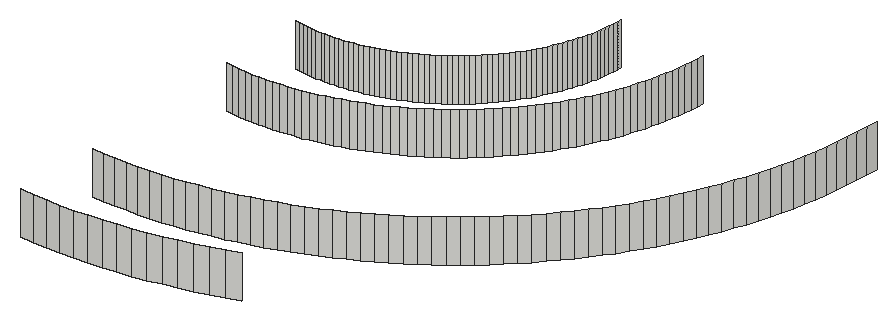
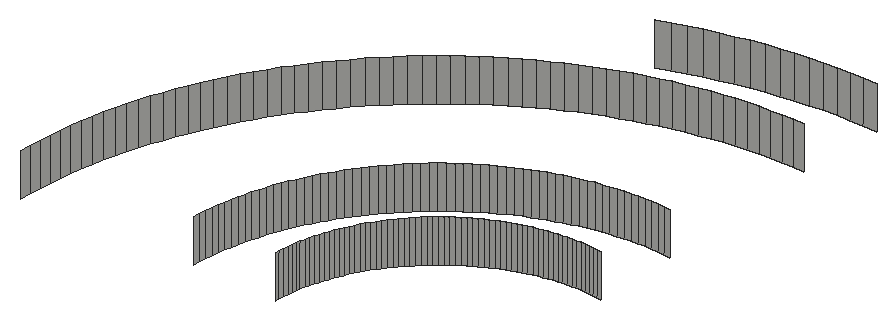
# SketchUp Ruby script. Lengths in inches.
U = 1.inch
M = Sketchup.active_model
def pt(a) = Geom::Point3d.new(a.map { |v| v * U })
def face(e, loops, mat)
  f = e.add_face(loops[0].map { |a| pt(a) })
  loops[1..].each { |l| e.add_face(l.map { |a| pt(a) }).erase! }
  f.material = f.back_material = mat if mat
  f
end
# faces: each face lists its corners as indices into pts; further lists are holes
def faces(e, pts, list, mat = nil) = list.each { |f| face(e, (f[0].is_a?(Array) ? f : [f]).map { |l| l.map { |i| pts[i] } }, mat) }
# xy, xz, yz: faces in a plane at the given z, y or x. An outline is a flat list of corners, or four numbers for a rectangle; further outlines are holes
def ring(l) = l.size == 4 ? [[l[0], l[1]], [l[2], l[1]], [l[2], l[3]], [l[0], l[3]]] : l.each_slice(2).to_a
def flat(e, list, mat, &to3) = list.each { |f| face(e, (f[0].is_a?(Array) ? f : [f]).map { |l| ring(l).map { |u, v| to3.(u, v) } }, mat) }
def xy(e, z, list, mat = nil) = flat(e, list, mat) { |x, y| [x, y, z] }
def xz(e, y, list, mat = nil) = flat(e, list, mat) { |x, z| [x, y, z] }
def yz(e, x, list, mat = nil) = flat(e, list, mat) { |y, z| [x, y, z] }
def lines(e, pts, list) = list.each { |a, b| e.add_line(pt(pts[a]), pt(pts[b])) }
# prism: a flat outline (further loops are holes) pulled along v
def prism(e, loops, v, mat = nil)
  f = face(e, loops, mat); d = Geom::Vector3d.new(v.map { |x| x * U })
  f.pushpull(f.normal.samedirection?(d) ? d.length : -d.length)
end
def box(e, o, s, mat = nil) = prism(e, [[o, [o[0] + s[0], o[1], o[2]], [o[0] + s[0], o[1] + s[1], o[2]], [o[0], o[1] + s[1], o[2]]]], [0, 0, s[2]], mat)
def at(x, y, z, deg = 0) = Geom::Transformation.translation(pt([x, y, z])) * Geom::Transformation.rotation(ORIGIN, Z_AXIS, deg.degrees)
def axes(o, x, y, z) = Geom::Transformation.new([*x, 0, *y, 0, *z, 0, *pt(o).to_a, 1])
def part(name) = M.definitions.add(name)
# library, detail: a bought-in or finely detailed component or shape, given as its bounding box
def library(name, o, s) = part(name).tap { |d| box(d.entities, o, s) }
def detail(e, o, s) = box(e.add_group.entities, o, s)
def put(e, d, t, mat = nil) = e.add_instance(d, t).tap { |i| i.material = mat if mat }
def group(e, t, mat = nil) = e.add_group.tap { |g| g.transformation = t; g.material = mat if mat }.entities
root = M.entities
xz(root,301.26,[[905.35,111.3125,905.98,117.3125],[905.98,111.3125,906.61,117.3125]])
p = [[904.09,253.28,117.3125],[902.21,253.35,117.3125],[902.21,253.35,111.3125],[904.09,253.28,111.3125],[905.98,253.26,117.3125],[905.98,253.26,111.3125],
  [907.86,253.28,117.3125],[907.86,253.28,111.3125],[909.75,253.35,117.3125],[909.75,253.35,111.3125],[911.63,253.48,117.3125],[911.63,253.48,111.3125],
  [913.5,253.65,117.3125],[913.5,253.65,111.3125],[915.375,253.87,117.3125],[915.375,253.87,111.3125],[917.24,254.14,117.3125],[917.24,254.14,111.3125],
  [919.1,254.46,117.3125],[919.1,254.46,111.3125],[920.95,254.83,117.3125],[920.95,254.83,111.3125],[922.79,255.25,117.3125],[922.79,255.25,111.3125],
  [924.61,255.71,117.3125],[924.61,255.71,111.3125],[926.43,256.22,117.3125],[926.43,256.22,111.3125],[928.23,256.78,117.3125],[928.23,256.78,111.3125],
  [930.01,257.39,117.3125],[930.01,257.39,111.3125],[902.84,265.34,117.3125],[904.41,265.28,117.3125],[904.41,265.28,111.3125],[902.84,265.34,111.3125],
  [905.98,265.26,117.3125],[905.98,265.26,111.3125],[907.55,265.28,117.3125],[907.55,265.28,111.3125],[909.12,265.34,117.3125],[909.12,265.34,111.3125],
  [910.6875,265.44,117.3125],[910.6875,265.44,111.3125],[912.25,265.58,117.3125],[912.25,265.58,111.3125],[913.81,265.77,117.3125],[913.81,265.77,111.3125],
  [915.36,265.99,117.3125],[915.36,265.99,111.3125],[916.91,266.26,117.3125],[916.91,266.26,111.3125],[918.45,266.57,117.3125],[918.45,266.57,111.3125],
  [919.99,266.91,117.3125],[919.99,266.91,111.3125],[921.51,267.3,117.3125],[921.51,267.3,111.3125],[923.02,267.73,117.3125],[923.02,267.73,111.3125],
  [924.52,268.19,117.3125],[924.52,268.19,111.3125],[926.01,268.7,117.3125],[926.01,268.7,111.3125],[927.48,269.24,117.3125],[927.48,269.24,111.3125],
  [928.94,269.82,117.3125],[928.94,269.82,111.3125],[930.38,270.44,117.3125],[930.38,270.44,111.3125],[931.81,271.1,117.3125],[931.81,271.1,111.3125],
  [933.22,271.8,117.3125],[933.22,271.8,111.3125],[934.61,272.53,117.3125],[934.61,272.53,111.3125],[935.98,273.29,117.3125],[935.98,273.29,111.3125],
  [937.33,274.1,117.3125],[937.33,274.1,111.3125],[938.66,274.9375,117.3125],[938.66,274.9375,111.3125],[939.96,275.81,117.3125],[939.96,275.81,111.3125],
  [941.25,276.72,117.3125],[941.25,276.72,111.3125],[942.5,277.66,117.3125],[942.5,277.66,111.3125],[943.74,278.63,117.3125],[943.74,278.63,111.3125],
  [944.95,279.63,117.3125],[944.95,279.63,111.3125],[946.125,280.67,117.3125],[946.125,280.67,111.3125],[947.28,281.73,117.3125],[947.28,281.73,111.3125],
  [948.41,282.83,117.3125],[948.41,282.83,111.3125],[949.5,283.95,117.3125],[949.5,283.95,111.3125],[950.57,285.11,117.3125],[950.57,285.11,111.3125],
  [951.6,286.29,117.3125],[951.6,286.29,111.3125],[952.61,287.5,117.3125],[952.61,287.5,111.3125],[953.58,288.73,117.3125],[953.58,288.73,111.3125],
  [954.52,289.99,117.3125],[954.52,289.99,111.3125],[904.09,289.31,117.3125],[903.15,289.37,117.3125],[903.15,289.37,111.3125],[904.09,289.31,111.3125],
  [905.04,289.27,117.3125],[905.04,289.27,111.3125],[905.98,289.26,117.3125],[905.98,289.26,111.3125],[906.92,289.27,117.3125],[906.92,289.27,111.3125],
  [907.86,289.31,117.3125],[907.86,289.31,111.3125],[908.8,289.37,117.3125],[908.8,289.37,111.3125],[902.22,289.45,117.3125],[902.22,289.45,111.3125],
  [909.74,289.45,117.3125],[909.74,289.45,111.3125],[910.68,289.5625,117.3125],[910.68,289.5625,111.3125],[911.61,289.7,117.3125],[911.61,289.7,111.3125],
  [912.54,289.86,117.3125],[912.54,289.86,111.3125],[913.46,290.04,117.3125],[913.46,290.04,111.3125],[914.38,290.25,117.3125],[914.38,290.25,111.3125],
  [955.43,291.27,117.3125],[955.43,291.27,111.3125],[915.3,290.48,117.3125],[915.3,290.48,111.3125],[916.2,290.74,117.3125],[916.2,290.74,111.3125],
  [917.1,291.02,117.3125],[917.1,291.02,111.3125],[918,291.32,117.3125],[918,291.32,111.3125],[918.88,291.65,117.3125],[918.88,291.65,111.3125],
  [956.3,292.58,117.3125],[956.3,292.58,111.3125],[919.76,292,117.3125],[919.76,292,111.3125],[920.62,292.37,117.3125],[920.62,292.37,111.3125],
  [921.48,292.76,117.3125],[921.48,292.76,111.3125],[957.14,293.91,117.3125],[957.14,293.91,111.3125],[922.32,293.18,117.3125],[922.32,293.18,111.3125],
  [923.16,293.62,117.3125],[923.16,293.62,111.3125],[923.98,294.08,117.3125],[923.98,294.08,111.3125],[957.94,295.26,117.3125],[957.94,295.26,111.3125],
  [924.79,294.5625,117.3125],[924.79,294.5625,111.3125],[925.59,295.0625,117.3125],[925.59,295.0625,111.3125],[926.37,295.59,117.3125],[926.37,295.59,111.3125],
  [958.71,296.625,117.3125],[958.71,296.625,111.3125],[927.14,296.13,117.3125],[927.14,296.13,111.3125],[927.89,296.7,117.3125],[927.89,296.7,111.3125],
  [959.4375,298.02,117.3125],[959.4375,298.02,111.3125],[928.63,297.28,117.3125],[928.63,297.28,111.3125],[929.36,297.88,117.3125],[929.36,297.88,111.3125],
  [930.07,298.5,117.3125],[930.07,298.5,111.3125],[960.13,299.43,117.3125],[960.13,299.43,111.3125],[930.76,299.14,117.3125],[930.76,299.14,111.3125],
  [931.43,299.8,117.3125],[931.43,299.8,111.3125],[960.79,300.85,117.3125],[960.79,300.85,111.3125],[932.09,300.48,117.3125],[932.09,300.48,111.3125],
  [932.73,301.17,117.3125],[932.73,301.17,111.3125],[961.41,302.3,117.3125],[961.41,302.3,111.3125],[933.35,301.875,117.3125],[933.35,301.875,111.3125],
  [903.47,301.39,117.3125],[904.1,301.33,117.3125],[904.1,301.33,111.3125],[903.47,301.39,111.3125],[904.72,301.29,117.3125],[904.72,301.29,111.3125],
  [905.35,301.26,117.3125],[905.35,301.26,111.3125],[906.61,301.26,117.3125],[907.23,301.29,117.3125],[907.23,301.29,111.3125],[906.61,301.26,111.3125],
  [907.86,301.33,117.3125],[907.86,301.33,111.3125],[908.49,301.39,117.3125],[908.49,301.39,111.3125],[902.85,301.46,117.3125],[902.85,301.46,111.3125],
  [909.11,301.46,117.3125],[909.11,301.46,111.3125],[902.22,301.55,117.3125],[902.22,301.55,111.3125],[909.73,301.55,117.3125],[909.73,301.55,111.3125],
  [910.35,301.66,117.3125],[910.35,301.66,111.3125],[910.97,301.78,117.3125],[910.97,301.78,111.3125],[911.58,301.92,117.3125],[911.58,301.92,111.3125],
  [912.19,302.07,117.3125],[912.19,302.07,111.3125],[933.96,302.6,117.3125],[933.96,302.6,111.3125],[912.8,302.24,117.3125],[912.8,302.24,111.3125],
  [913.4,302.43,117.3125],[913.4,302.43,111.3125],[961.99,303.75,117.3125],[961.99,303.75,111.3125],[913.99,302.63,117.3125],[913.99,302.63,111.3125],
  [914.58,302.85,117.3125],[914.58,302.85,111.3125],[934.54,303.34,117.3125],[934.54,303.34,111.3125],[915.16,303.08,117.3125],[915.16,303.08,111.3125],
  [915.74,303.33,117.3125],[915.74,303.33,111.3125],[916.3125,303.59,117.3125],[916.3125,303.59,111.3125],[935.1,304.1,117.3125],[935.1,304.1,111.3125],
  [916.875,303.87,117.3125],[916.875,303.87,111.3125],[962.54,305.23,117.3125],[962.54,305.23,111.3125],[917.43,304.16,117.3125],[917.43,304.16,111.3125],
  [935.65,304.87,117.3125],[935.65,304.87,111.3125],[917.98,304.47,117.3125],[917.98,304.47,111.3125],[918.52,304.79,117.3125],[918.52,304.79,111.3125],
  [919.05,305.13,117.3125],[919.05,305.13,111.3125],[936.17,305.65,117.3125],[936.17,305.65,111.3125],[919.57,305.48,117.3125],[919.57,305.48,111.3125],
  [963.04,306.72,117.3125],[963.04,306.72,111.3125],[920.09,305.84,117.3125],[920.09,305.84,111.3125],[936.67,306.45,117.3125],[936.67,306.45,111.3125],
  [920.59,306.22,117.3125],[920.59,306.22,111.3125],[921.08,306.6,117.3125],[921.08,306.6,111.3125],[937.16,307.26,117.3125],[937.16,307.26,111.3125],
  [921.57,307.01,117.3125],[921.57,307.01,111.3125],[963.51,308.22,117.3125],[963.51,308.22,111.3125],[922.04,307.42,117.3125],[922.04,307.42,111.3125],
  [937.62,308.08,117.3125],[937.62,308.08,111.3125],[922.5,307.85,117.3125],[922.5,307.85,111.3125],[922.95,308.29,117.3125],[922.95,308.29,111.3125],
  [938.05,308.91,117.3125],[938.05,308.91,111.3125],[963.93,309.73,117.3125],[963.93,309.73,111.3125],[923.39,308.74,117.3125],[923.39,308.74,111.3125],
  [923.8125,309.2,117.3125],[923.8125,309.2,111.3125],[938.47,309.76,117.3125],[938.47,309.76,111.3125],[924.23,309.67,117.3125],[924.23,309.67,111.3125],
  [924.63,310.15,117.3125],[924.63,310.15,111.3125],[964.32,311.25,117.3125],[964.32,311.25,111.3125],[938.87,310.61,117.3125],[938.87,310.61,111.3125],
  [925.02,310.65,117.3125],[925.02,310.65,111.3125],[925.4,311.15,117.3125],[925.4,311.15,111.3125],[939.24,311.48,117.3125],[939.24,311.48,111.3125],
  [925.76,311.66,117.3125],[925.76,311.66,111.3125],[964.67,312.78,117.3125],[964.67,312.78,111.3125],[939.59,312.35,117.3125],[939.59,312.35,111.3125],
  [926.11,312.18,117.3125],[926.11,312.18,111.3125],[926.44,312.72,117.3125],[926.44,312.72,111.3125],[939.91,313.24,117.3125],[939.91,313.24,111.3125],
  [926.76,313.26,117.3125],[926.76,313.26,111.3125],[964.97,314.32,117.3125],[964.97,314.32,111.3125],[940.22,314.13,117.3125],[940.22,314.13,111.3125],
  [927.07,313.8,117.3125],[927.07,313.8,111.3125],[927.36,314.36,117.3125],[927.36,314.36,111.3125],[940.5,315.03,117.3125],[940.5,315.03,111.3125],
  [965.24,315.87,117.3125],[965.24,315.87,111.3125],[927.64,314.92,117.3125],[927.64,314.92,111.3125],[927.9,315.49,117.3125],[927.9,315.49,111.3125],
  [940.75,315.9375,117.3125],[940.75,315.9375,111.3125],[928.15,316.07,117.3125],[928.15,316.07,111.3125],[940.98,316.85,117.3125],[940.98,316.85,111.3125],
  [965.47,317.42,117.3125],[965.47,317.42,111.3125],[928.38,316.66,117.3125],[928.38,316.66,111.3125],[928.6,317.24,117.3125],[928.6,317.24,111.3125],
  [941.19,317.77,117.3125],[941.19,317.77,111.3125],[928.8,317.84,117.3125],[928.8,317.84,111.3125],[965.65,318.98,117.3125],[965.65,318.98,111.3125],
  [928.99,318.44,117.3125],[928.99,318.44,111.3125],[941.375,318.7,117.3125],[941.375,318.7,111.3125],[929.16,319.04,117.3125],[929.16,319.04,111.3125],
  [941.54,319.625,117.3125],[941.54,319.625,111.3125],[929.32,319.65,117.3125],[929.32,319.65,111.3125],[965.79,320.55,117.3125],[965.79,320.55,111.3125],
  [941.67,320.56,117.3125],[941.67,320.56,111.3125],[929.45,320.27,117.3125],[929.45,320.27,111.3125],[929.58,320.88,117.3125],[929.58,320.88,111.3125],
  [965.9,322.12,117.3125],[965.9,322.12,111.3125],[941.78,321.49,117.3125],[941.78,321.49,111.3125],[929.68,321.5,117.3125],[929.68,321.5,111.3125],
  [929.77,322.125,117.3125],[929.77,322.125,111.3125],[941.87,322.43,117.3125],[941.87,322.43,111.3125],[929.85,322.75,117.3125],[929.85,322.75,111.3125],
  [965.96,323.6875,117.3125],[965.96,323.6875,111.3125],[941.93,323.37,117.3125],[941.93,323.37,111.3125],[929.9,323.375,117.3125],[929.9,323.375,111.3125],
  [929.95,324,117.3125],[929.95,324,111.3125]]
faces(root,p,[[0,1,2,3],[4,0,3,5],[6,4,5,7],[8,6,7,9],[10,8,9,11],[12,10,11,13],[14,12,13,15],[16,14,15,17],
  [18,16,17,19],[20,18,19,21],[22,20,21,23],[24,22,23,25],[26,24,25,27],[28,26,27,29],[30,28,29,31],[32,33,34,35],
  [33,36,37,34],[36,38,39,37],[38,40,41,39],[40,42,43,41],[42,44,45,43],[44,46,47,45],[46,48,49,47],[48,50,51,49],
  [50,52,53,51],[52,54,55,53],[54,56,57,55],[56,58,59,57],[58,60,61,59],[60,62,63,61],[62,64,65,63],[64,66,67,65],
  [66,68,69,67],[68,70,71,69],[70,72,73,71],[72,74,75,73],[74,76,77,75],[76,78,79,77],[78,80,81,79],[80,82,83,81],
  [82,84,85,83],[84,86,87,85],[86,88,89,87],[88,90,91,89],[90,92,93,91],[92,94,95,93],[94,96,97,95],[96,98,99,97],
  [98,100,101,99],[100,102,103,101],[102,104,105,103],[104,106,107,105],[106,108,109,107],[110,111,112,113],[114,110,113,115],[116,114,115,117],
  [118,116,117,119],[120,118,119,121],[122,120,121,123],[111,124,125,112],[126,122,123,127],[128,126,127,129],[130,128,129,131],[132,130,131,133],
  [134,132,133,135],[136,134,135,137],[108,138,139,109],[140,136,137,141],[142,140,141,143],[144,142,143,145],[146,144,145,147],[148,146,147,149],
  [138,150,151,139],[152,148,149,153],[154,152,153,155],[156,154,155,157],[150,158,159,151],[160,156,157,161],[162,160,161,163],[164,162,163,165],
  [158,166,167,159],[168,164,165,169],[170,168,169,171],[172,170,171,173],[166,174,175,167],[176,172,173,177],[178,176,177,179],[174,180,181,175],
  [182,178,179,183],[184,182,183,185],[186,184,185,187],[180,188,189,181],[190,186,187,191],[192,190,191,193],[188,194,195,189],[196,192,193,197],
  [198,196,197,199],[194,200,201,195],[202,198,199,203],[204,205,206,207],[205,208,209,206],[208,210,211,209],[212,213,214,215],[213,216,217,214],
  [216,218,219,217],[220,204,207,221],[218,222,223,219],[224,220,221,225],[222,226,227,223],[226,228,229,227],[228,230,231,229],[230,232,233,231],
  [232,234,235,233],[236,202,203,237],[234,238,239,235],[238,240,241,239],[200,242,243,201],[240,244,245,241],[244,246,247,245],[248,236,237,249],
  [246,250,251,247],[250,252,253,251],[252,254,255,253],[256,248,249,257],[254,258,259,255],[242,260,261,243],[258,262,263,259],[264,256,257,265],
  [262,266,267,263],[266,268,269,267],[268,270,271,269],[272,264,265,273],[270,274,275,271],[260,276,277,261],[274,278,279,275],[280,272,273,281],
  [278,282,283,279],[282,284,285,283],[286,280,281,287],[284,288,289,285],[276,290,291,277],[288,292,293,289],[294,286,287,295],[292,296,297,293],
  [296,298,299,297],[300,294,295,301],[290,302,303,291],[298,304,305,299],[304,306,307,305],[308,300,301,309],[306,310,311,307],[310,312,313,311],
  [302,314,315,303],[316,308,309,317],[312,318,319,313],[318,320,321,319],[322,316,317,323],[320,324,325,321],[314,326,327,315],[328,322,323,329],
  [324,330,331,325],[330,332,333,331],[334,328,329,335],[332,336,337,333],[326,338,339,327],[340,334,335,341],[336,342,343,337],[342,344,345,343],
  [346,340,341,347],[338,348,349,339],[344,350,351,345],[350,352,353,351],[354,346,347,355],[352,356,357,353],[358,354,355,359],[348,360,361,349],
  [356,362,363,357],[362,364,365,363],[366,358,359,367],[364,368,369,365],[360,370,371,361],[368,372,373,369],[374,366,367,375],[372,376,377,373],
  [378,374,375,379],[376,380,381,377],[370,382,383,371],[384,378,379,385],[380,386,387,381],[386,388,389,387],[382,390,391,383],[392,384,385,393],
  [388,394,395,389],[394,396,397,395],[398,392,393,399],[396,400,401,397],[390,402,403,391],[404,398,399,405],[400,406,407,401],[406,408,409,407]])
